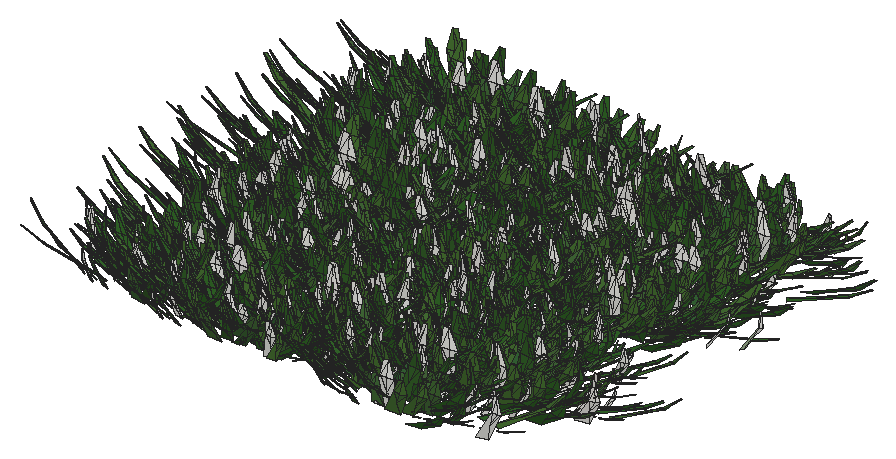
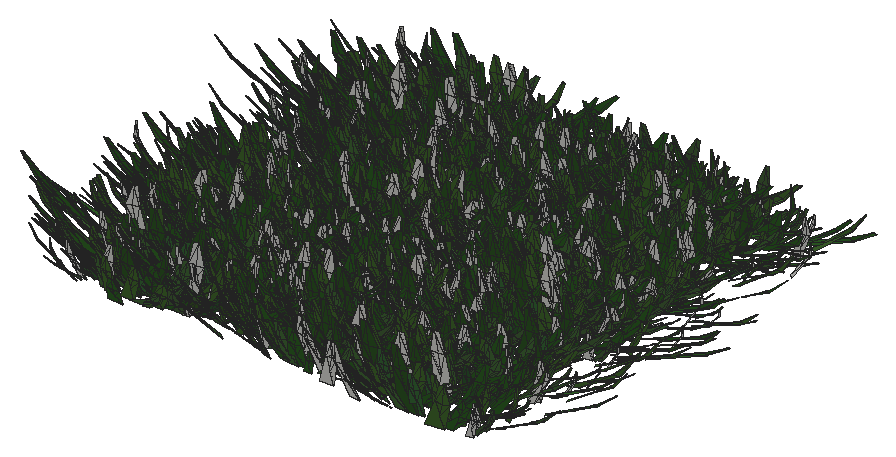
# SketchUp Ruby script. Lengths in inches.
U = 1.inch
M = Sketchup.active_model
def pt(a) = Geom::Point3d.new(a.map { |v| v * U })
def face(e, loops, mat)
  f = e.add_face(loops[0].map { |a| pt(a) })
  loops[1..].each { |l| e.add_face(l.map { |a| pt(a) }).erase! }
  f.material = f.back_material = mat if mat
  f
end
# faces: each face lists its corners as indices into pts; further lists are holes
def faces(e, pts, list, mat = nil) = list.each { |f| face(e, (f[0].is_a?(Array) ? f : [f]).map { |l| l.map { |i| pts[i] } }, mat) }
# xy, xz, yz: faces in a plane at the given z, y or x. An outline is a flat list of corners, or four numbers for a rectangle; further outlines are holes
def ring(l) = l.size == 4 ? [[l[0], l[1]], [l[2], l[1]], [l[2], l[3]], [l[0], l[3]]] : l.each_slice(2).to_a
def flat(e, list, mat, &to3) = list.each { |f| face(e, (f[0].is_a?(Array) ? f : [f]).map { |l| ring(l).map { |u, v| to3.(u, v) } }, mat) }
def xy(e, z, list, mat = nil) = flat(e, list, mat) { |x, y| [x, y, z] }
def xz(e, y, list, mat = nil) = flat(e, list, mat) { |x, z| [x, y, z] }
def yz(e, x, list, mat = nil) = flat(e, list, mat) { |y, z| [x, y, z] }
def lines(e, pts, list) = list.each { |a, b| e.add_line(pt(pts[a]), pt(pts[b])) }
# prism: a flat outline (further loops are holes) pulled along v
def prism(e, loops, v, mat = nil)
  f = face(e, loops, mat); d = Geom::Vector3d.new(v.map { |x| x * U })
  f.pushpull(f.normal.samedirection?(d) ? d.length : -d.length)
end
def box(e, o, s, mat = nil) = prism(e, [[o, [o[0] + s[0], o[1], o[2]], [o[0] + s[0], o[1] + s[1], o[2]], [o[0], o[1] + s[1], o[2]]]], [0, 0, s[2]], mat)
def at(x, y, z, deg = 0) = Geom::Transformation.translation(pt([x, y, z])) * Geom::Transformation.rotation(ORIGIN, Z_AXIS, deg.degrees)
def axes(o, x, y, z) = Geom::Transformation.new([*x, 0, *y, 0, *z, 0, *pt(o).to_a, 1])
def part(name) = M.definitions.add(name)
# library, detail: a bought-in or finely detailed component or shape, given as its bounding box
def library(name, o, s) = part(name).tap { |d| box(d.entities, o, s) }
def detail(e, o, s) = box(e.add_group.entities, o, s)
def put(e, d, t, mat = nil) = e.add_instance(d, t).tap { |i| i.material = mat if mat }
def group(e, t, mat = nil) = e.add_group.tap { |g| g.transformation = t; g.material = mat if mat }.entities
root = M.entities
M.materials.add("Material10").color = [48, 100, 38]
M.materials.add("Material3").color = [68, 110, 58]
M.materials.add("Material4").color = [48, 90, 38]
M.materials.add("Material5").color = [68, 110, 48]
M.materials.add("Material6").color = [48, 90, 48]
M.materials.add("Material7").color = [58, 110, 58]
M.materials.add("Material8").color = [58, 90, 38]
M.materials.add("Material9").color = [68, 100, 58]
c1 = part("grass00")
p = [[-0.6875,0.15,0],[-0.56,0.08,5.52],[-0.04,0.03,2.76],[0.48,-0.02,0],[0.35,-0.02,5.52],[-0.1,-0.14,5.52],
  [-0.12,0.65,8.37],[-0.42,0.65,8.37]]
faces(c1.entities,p,[[0,1,2,3],[3,2,4],[1,5,2],[5,4,2],[1,6,5],[4,5,6],[7,6,1]])
c2 = part("Group16\#1")
put(c2.entities,c1,axes([1.44,-0.61,-0.01],[0.05352,0.12609,0],[-0.10704,0.04543,0.07239],[0.06664,-0.02828,0.11628]),"Material6")
put(c2.entities,c1,axes([0.76,-0.15,-0.01],[0.04676,0.24062,0],[-0.23162,0.04501,0.06642],[0.0652,-0.01267,0.23595]),"Material3")
put(c2.entities,c1,axes([0.79,0.01,-0.01],[-0.00606,0.34651,0],[-0.34381,-0.00602,0.0432],[0.04319,0.00076,0.34386]))
put(c2.entities,c1,axes([1,0.23,-0.01],[-0.07192,0.31144,0],[-0.28722,-0.06632,0.1236],[0.12043,0.02781,0.29478]),"Material5")
put(c2.entities,c1,axes([1.66,0.77,-0.01],[-0.13828,0.29651,0],[-0.21551,-0.1005,0.22471],[0.20365,0.09498,0.23779]),"Material10")
put(c2.entities,c1,axes([0.6875,0.52,-0.01],[-0.18126,0.24051,0],[-0.22746,-0.17142,0.09788],[0.07817,0.05891,0.28481]),"Material5")
put(c2.entities,c1,axes([0.68,0.78,-0.01],[-0.215,0.18688,0],[-0.12385,-0.14248,0.21334],[0.13995,0.16101,0.18878]),"Material3")
put(c2.entities,c1,axes([0.56,1,-0.01],[-0.13756,0.07624,0],[-0.06159,-0.11112,0.0927],[0.04494,0.08108,0.12705]),"Material5")
put(c2.entities,c1,axes([0.2,0.64,-0.01],[-0.23729,0.07254,0],[-0.05711,-0.18681,0.153],[0.04473,0.14632,0.19535]),"Material10")
put(c2.entities,c1,axes([0.0625,0.72,-0.01],[-0.28874,0.02525,0],[-0.02179,-0.24916,0.14647],[0.01276,0.14591,0.25012]),"Material3")
put(c2.entities,c1,axes([-0.08,0.62,-0.01],[-0.34089,-0.04187,0],[0.03255,-0.26504,0.216],[-0.02633,0.21439,0.26703]),"Material10")
put(c2.entities,c1,axes([-0.34,0.98,-0.01],[-0.14314,-0.0493,0],[0.04397,-0.12769,0.06843],[-0.02228,0.0647,0.13505]),"Material10")
put(c2.entities,c1,axes([-0.87,1.45,-0.01],[-0.23488,-0.14114,0],[0.13761,-0.22901,0.06087],[-0.03135,0.05217,0.26717]))
put(c2.entities,c1,axes([-0.72,0.77,-0.01],[-0.14208,-0.13251,0],[0.07209,-0.0773,0.16301],[-0.11118,0.11922,0.1057]),"Material10")
put(c2.entities,c1,axes([-0.62,0.43,-0.01],[-0.14845,-0.21203,0],[0.18654,-0.13061,0.12304],[-0.10079,0.07057,0.22772]),"Material3")
put(c2.entities,c1,axes([-0.68,0.29,-0.01],[-0.13639,-0.32136,0],[0.31723,-0.13464,0.05579],[-0.05136,0.0218,0.34462]),"Material4")
put(c2.entities,c1,axes([-0.64,0.125,-0.01],[-0.0458,-0.23569,0],[0.22124,-0.043,0.08276],[-0.08124,0.01579,0.22538]),"Material7")
put(c2.entities,c1,axes([-1.6,-0.03,-0.01],[0.00576,-0.32897,0],[0.27526,0.00482,0.18018],[-0.18015,-0.00315,0.2753]),"Material5")
put(c2.entities,c1,axes([-1.36,-0.31,-0.01],[0.05718,-0.24765,0],[0.18172,0.04196,0.17267],[-0.16825,-0.03885,0.1865]),"Material10")
put(c2.entities,c1,axes([-1.54,-0.72,-0.01],[0.06537,-0.14017,0],[0.13555,0.06321,0.03939],[-0.0357,-0.01665,0.14956]))
put(c2.entities,c1,axes([-1.19,-0.9,-0.01],[0.09597,-0.12735,0],[0.11214,0.08451,0.07557],[-0.06035,-0.04548,0.14042]),"Material9")
put(c2.entities,c1,axes([-0.47,-0.54,-0.01],[0.11588,-0.10072,0],[0.0618,0.0711,0.12124],[-0.07953,-0.0915,0.0942]))
put(c2.entities,c1,axes([-0.47,-0.84,-0.01],[0.11927,-0.0661,0],[0.06603,0.11913,0.00646],[-0.00313,-0.00565,0.13621]),"Material5")
put(c2.entities,c1,axes([-0.38,-1.24,-0.01],[0.28037,-0.08571,0],[0.0618,0.20215,0.20315],[-0.05939,-0.19428,0.21139]),"Material9")
put(c2.entities,c1,axes([-0.06,-0.66,-0.01],[0.22719,-0.01987,0],[0.01247,0.14255,0.17758],[-0.01547,-0.17691,0.1431]),"Material8")
put(c2.entities,c1,axes([0.11,-0.89,-0.01],[0.14882,0.01828,0],[-0.01058,0.08611,0.12229],[0.01491,-0.12138,0.08676]),"Material6")
put(c2.entities,c1,axes([0.25,-0.72,-0.01],[0.20481,0.07053,0],[-0.06206,0.18022,0.10291],[0.03351,-0.0973,0.1906]),"Material6")
put(c2.entities,c1,axes([0.85,-1.42,-0.01],[0.16481,0.09904,0],[-0.09472,0.15762,0.05616],[0.02893,-0.04814,0.18389]),"Material5")
put(c2.entities,c1,axes([1.01,-1.09,-0.01],[0.21858,0.20385,0],[-0.17495,0.1876,0.15339],[0.10462,-0.11218,0.25652]),"Material10")
put(c2.entities,c1,axes([1.01,-0.71,-0.01],[0.08733,0.12473,0],[-0.06445,0.04512,0.13037],[0.1068,-0.07477,0.07867]),"Material6")
c3 = part("Group15\#1")
put(c3.entities,c2,at(0,0,0))
c4 = part("3darcstudiotree_grass00\#1")
put(c4.entities,c3,at(0,0,0))
put(root,c4,axes([60.36,24.12,7.6],[4.14217,-0.13896,0],[0.55231,1.029,-0.04419],[0.03401,0.06336,1.50171]))
put(root,c4,axes([61.51,38.26,7.6],[-3.78089,0.19176,0],[-0.79047,-0.97412,-0.01756],[-0.02482,-0.03059,1.76676]))
put(root,c4,axes([60.24,5.63,7.6],[3.46429,0.31864,0],[-1.65951,1.12765,-0.05896],[-0.1317,0.08949,1.94308]))
put(root,c4,axes([61.51,41.64,7.6],[0.85917,-1.09149,0],[4.23857,0.20853,-0.05061],[0.35882,0.01765,1.95081]))
put(root,c4,axes([62.11,26.89,7.6],[-4.66063,0.03187,0],[-0.11925,-1.09003,-0.04984],[-0.00747,-0.06831,1.49526]))
put(root,c4,axes([62.08,27.74,7.6],[0.72703,-1.03791,0],[5.00906,0.2193,-0.04237],[0.25355,0.0111,1.93074]))
put(root,c4,axes([61.48,22.57,7.6],[-2.37788,0.70827,0],[-3.16948,-0.66506,-0.02769],[-0.12287,-0.02578,1.49833]))
put(root,c4,axes([61.58,17.12,7.6],[-1.33257,1.11257,0],[-3.55566,-0.26617,-0.04102],[-0.28293,-0.02118,1.67021]))
put(root,c4,axes([62.17,16.2,7.6],[-3.55507,0.28812,0],[-1.24707,-0.96172,-0.02033],[-0.04772,-0.0368,1.92362]))
put(root,c4,axes([61.1875,35.42,7.6],[4.13598,0.19347,0],[-0.75584,1.00989,-0.00485],[-0.0061,0.00815,1.75633]))
put(root,c4,axes([61.05,9.8,7.6],[0.77095,1.02886,0],[-4.76297,0.22306,-0.00799],[-0.0391,0.00183,1.50733]))
put(root,c4,axes([61.85,19.33,7.6],[4.78466,-0.38044,0],[1.18012,0.92761,-0.00335],[0.00607,0.00477,1.45436]))
put(root,c4,axes([62.82,43.23,7.6],[1.77249,-0.83828,0],[4.36469,0.5768,-0.05061],[0.28357,0.03747,1.95538]))
put(root,c4,axes([63.67,6.61,7.6],[-4.81545,-0.2901,0],[1.06341,-1.10323,-0.03666],[0.0394,-0.04088,1.30149]))
put(root,c4,axes([64,11.27,7.6],[-3.36311,-0.90745,0],[3.5657,-0.82593,-0.02123],[0.07378,-0.01709,1.43939]))
put(root,c4,axes([62.4,29.69,7.6],[4.34926,-0.09263,0],[0.33262,0.97608,-0.01096],[0.00735,0.02158,1.93666]))
put(root,c4,axes([63.82,34.02,7.6],[1.03751,-0.98763,0],[4.08479,0.26819,-0.03356],[0.19811,0.01301,1.61101]))
put(root,c4,axes([62.71,12.97,7.6],[4.36652,-0.10456,0],[0.38952,1.01663,-0.02913],[0.02165,0.05651,1.9903]))
put(root,c4,axes([64.2,25.04,7.6],[0.12365,-1.27532,0],[4.95988,0.03006,-0.04883],[0.25094,0.00152,1.59403]))
put(root,c4,axes([62.38,20.43,7.6],[1.52464,0.86954,0],[-4.15594,0.45544,-0.01361],[-0.07039,0.00771,1.60179]))
put(root,c4,axes([63.23,32.51,7.6],[4.76541,-0.43818,0],[1.55968,1.06014,-0.01984],[0.0463,0.03147,1.90869]))
put(root,c4,axes([63.68,36.97,7.6],[3.07982,0.93534,0],[-3.08003,0.63386,-0.01155],[-0.0607,0.01249,1.69697]))
put(root,c4,axes([66.08,18.09,7.6],[-3.49123,-0.27922,0],[1.51464,-1.18364,-0.00535],[0.00882,-0.00689,1.67969]))
put(root,c4,axes([66.24,24,7.6],[0.13314,-1.12565,0],[4.81374,0.03558,-0.0158],[0.0905,0.00067,1.72451]))
put(root,c4,axes([66.53,10.14,7.6],[0.0625,-0.92457,0],[5.11457,0.02161,-0.02351],[0.11863,0.0005,1.61343]))
put(root,c4,axes([65.87,15.59,7.6],[2.8016,-0.76743,0],[3.52577,0.80446,-0.03913],[0.15024,0.03428,1.55084]))
put(root,c4,axes([66.61,27.98,7.6],[-5.10128,0.24176,0],[-0.82054,-1.08211,-0.04366],[-0.05047,-0.06656,1.70895]))
put(root,c4,axes([66.96,22.38,7.6],[-4.96044,-0.06591,0],[0.25075,-1.17948,-0.02618],[0.00816,-0.03838,1.73378]))
put(root,c4,axes([67.33,35.67,7.6],[-3.94461,-0.5014,0],[1.7984,-0.88427,-0.05096],[0.14967,-0.07359,1.60728]))
put(root,c4,axes([65.98,34.6,7.6],[3.7762,-0.18672,0],[0.72842,0.92072,-0.00259],[0.00364,0.0046,1.70099]))
put(root,c4,axes([66.33,31.47,7.6],[3.67314,-0.43874,0],[1.76522,0.92366,-0.01719],[0.04935,0.02582,1.70421]))
put(root,c4,axes([67.75,39.09,7.6],[-3.93857,-0.30978,0],[1.37085,-1.08932,-0.00258],[0.00367,-0.00291,1.35273]))
put(root,c4,axes([68.09,11.4375,7.6],[-3.44755,-0.92992,0],[3.38069,-0.78334,-0.01903],[0.09302,-0.02155,1.91973]))
put(root,c4,axes([66.99,18.61,7.6],[-2.366,0.989,0],[-3.30831,-0.49466,-0.01081],[-0.05313,-0.00794,1.38013]))
put(root,c4,axes([67.5,41.79,7.6],[2.17212,-0.7546,0],[4.09706,0.73708,-0.05142],[0.26111,0.04697,1.97373]))
put(root,c4,axes([66.51,20.67,7.6],[2.16605,0.76484,0],[-3.80323,0.67318,-0.06047],[-0.22732,0.04024,1.34144]))
put(root,c4,axes([68.42,37.48,7.6],[-1.30769,-0.93335,0],[3.48924,-0.30554,-0.02961],[0.16247,-0.01423,1.34337]))
put(root,c4,axes([67.46,14.66,7.6],[-1.89044,1.0999,0],[-3.63234,-0.39019,-0.02574],[-0.12693,-0.01363,1.32606]))
put(root,c4,axes([67.45,26.95,7.6],[3.25343,-0.44268,0],[1.93711,0.88978,-0.04084],[0.14968,0.06875,1.94165]))
put(root,c4,axes([69.23,29.77,7.6],[-2.99003,-0.56506,0],[2.79267,-0.92359,-0.03674],[0.12403,-0.04102,1.62045]))
put(root,c4,axes([69.23,8.03,7.6],[-4.96013,0.01619,0],[-0.06304,-1.20724,-0.02897],[-0.0018,-0.03442,1.4344]))
put(root,c4,axes([67.97,39.8,7.6],[3.80777,-0.2002,0],[0.96857,1.15138,-0.04208],[0.03932,0.04675,1.3356]))
put(root,c4,axes([67.88,5.97,7.6],[3.481,0.74238,0],[-3.25262,0.95321,-0.05603],[-0.20851,0.06111,1.79617]))
put(root,c4,axes([69.37,13.11,7.6],[-3.23012,0.53983,0],[-2.03325,-0.76039,-0.00767],[-0.03049,-0.0114,1.63569]))
put(root,c4,axes([69.7,33.16,7.6],[1.70325,-1.05974,0],[4.66988,0.4691,-0.03894],[0.22464,0.02257,1.95573]))
put(root,c4,axes([69.53,25.52,7.6],[2.4144,-1.08588,0],[3.3917,0.47133,-0.02727],[0.14209,0.01975,1.44583]))
put(root,c4,axes([68.93,6.75,7.6],[4.57432,-0.02417,0],[0.10814,1.27933,-0.00824],[0.00087,0.0103,1.59977]))
put(root,c4,axes([69.38,4.33,7.6],[4.10387,0.33855,0],[-1.15114,0.87212,-0.0401],[-0.09251,0.07009,1.69032]))
put(root,c4,axes([71.99,29.92,7.6],[-4.98676,0.19311,0],[-0.7421,-1.19771,-0.03016],[-0.02479,-0.04002,1.62739]))
put(root,c4,axes([73.03,20.97,7.6],[-1.79404,-0.94481,0],[3.82512,-0.45395,-0.00409],[0.0193,-0.00229,1.3842]))
put(root,c4,axes([72.42,5.19,7.6],[-3.73442,0.23061,0],[-0.95038,-0.96187,-0.03348],[-0.04929,-0.04988,1.52035]))
put(root,c4,axes([72.89,21.68,7.6],[2.59296,-0.87117,0],[4.05566,0.75445,-0.00846],[0.02997,0.00558,1.39582]))
put(root,c4,axes([73.77,38.4,7.6],[-4.85,-0.22958,0],[0.83383,-1.10092,-0.02653],[0.02986,-0.03943,1.69452]))
put(root,c4,axes([73.76,16.42,7.6],[-3.94716,-0.15767,0],[0.6625,-1.03659,-0.01241],[0.00983,-0.01538,1.31731]))
put(root,c4,axes([72.55,24.99,7.6],[4.34642,-0.40872,0],[1.45862,0.96946,-0.01237],[0.03108,0.02066,1.84855]))
put(root,c4,axes([74.2,7.96,7.6],[-4.3345,-0.18054,0],[0.62418,-0.93658,-0.01531],[0.0191,-0.02866,1.80136]))
put(root,c4,axes([74.04,10.92,7.6],[1.02924,-1.1219,0],[3.76479,0.21587,-0.013],[0.10318,0.00592,1.96601]))
put(root,c4,axes([74.49,13.13,7.6],[-1.06084,-1.17828,0],[4.37174,-0.246,-0.03143],[0.16722,-0.00941,1.52743]))
put(root,c4,axes([74.82,28.58,7.6],[-1.72294,-1.06651,0],[4.16754,-0.42079,-0.01424],[0.06745,-0.00681,1.43479]))
put(root,c4,axes([74.66,39.85,7.6],[-3.78747,-0.21466,0],[0.95822,-1.0567,-0.03754],[0.05955,-0.06567,1.94323]))
put(root,c4,axes([74.34,14.06,7.6],[-0.48134,-1.10906,0],[3.87122,-0.10501,-0.05057],[0.36681,-0.00995,1.77563]))
put(root,c4,axes([73.23,23.59,7.6],[3.37993,0.45978,0],[-1.93327,0.88823,-0.04213],[-0.10808,0.04966,1.35679]))
put(root,c4,axes([74.55,10.36,7.6],[3.21509,-0.82009,0],[3.01925,0.73979,-0.0131],[0.0637,0.01561,1.79861]))
put(root,c4,axes([75.48,30.62,7.6],[-3.80165,-0.22525,0],[1.19413,-1.25962,-0.00987],[0.01044,-0.01102,1.48448]))
put(root,c4,axes([73.49,19.04,7.6],[3.93668,0.7746,0],[-2.90323,0.92217,-0.01986],[-0.08093,0.02571,1.93312]))
put(root,c4,axes([74.39,7.09,7.6],[-0.79276,1.18933,0],[-3.59183,-0.14964,-0.00349],[-0.02047,-0.00085,1.35435]))
put(root,c4,axes([74.4,43.01,7.6],[4.30418,0.00494,0],[-0.017,0.92497,-0.03904],[-0.00144,0.07818,1.85207]))
put(root,c4,axes([75.5,17,7.6],[2.16099,-1.18023,0],[3.73882,0.42786,-0.04178],[0.24002,0.02747,1.62381]))
put(root,c4,axes([74.5625,26.15,7.6],[3.61999,0.64217,0],[-2.78348,0.98067,-0.05586],[-0.16431,0.05789,1.52805]))
put(root,c4,axes([75.58,37.33,7.6],[3.39209,-0.30668,0],[1.53109,1.05845,-0.04794],[0.07887,0.05453,1.36124]))
put(root,c4,axes([76.4,36.27,7.6],[3.28078,-0.54762,0],[2.6685,0.99917,-0.03164],[0.11118,0.04163,1.90074]))
put(root,c4,axes([76,41.43,7.6],[4.6588,-0.38386,0],[1.34446,1.01982,-0.0158],[0.03633,0.02756,1.97161]))
put(root,c4,axes([75.625,34.56,7.6],[1.88884,1.20061,0],[-4.32214,0.42498,-0.01805],[-0.11016,0.01083,1.90362]))
put(root,c4,axes([76.23,32.34,7.6],[4.87019,-0.36873,0],[1.38522,1.1435,-0.03542],[0.04951,0.04087,1.44036]))
put(root,c4,axes([78.15,20.7,7.6],[-3.20652,-0.59771,0],[2.76266,-0.9263,-0.01853],[0.05834,-0.01956,1.52144]))
put(root,c4,axes([78.47,28.7,7.6],[-4.04993,-0.77594,0],[2.93522,-0.9575,-0.01589],[0.04448,-0.01451,1.38765]))
put(root,c4,axes([78.11,32.58,7.6],[-4.54229,0.0918,0],[-0.30554,-0.94485,-0.02584],[-0.01532,-0.04736,1.74304]))
put(root,c4,axes([77.99,37.32,7.6],[2.61594,-0.62324,0],[2.61447,0.68586,-0.03437],[0.16704,0.04382,1.66865]))
put(root,c4,axes([78.76,40.17,7.6],[0.42125,-1.19943,0],[4.10961,0.09021,-0.02351],[0.14993,0.00329,1.65028]))
put(root,c4,axes([78.09,17.46,7.6],[3.29935,0.67285,0],[-2.48006,0.76006,-0.0073],[-0.03648,0.01118,1.93831]))
put(root,c4,axes([80.25,41.24,7.6],[-4.60962,0.0959,0],[-0.32649,-0.98088,-0.01346],[-0.00781,-0.02346,1.72106]))
put(root,c4,axes([80.52,8.36,7.6],[-3.45897,-0.26737,0],[1.38281,-1.1181,-0.02785],[0.05102,-0.04126,1.81462]))
put(root,c4,axes([79.79,11.58,7.6],[-1.6569,0.8411,0],[-3.67968,-0.45304,-0.03193],[-0.19007,-0.0234,1.70102]))
put(root,c4,axes([81.03,16.01,7.6],[-4.11024,0.08918,0],[-0.31404,-0.9046,-0.03872],[-0.02635,-0.07591,1.78675]))
put(root,c4,axes([79.99,12.98,7.6],[3.52313,0.28357,0],[-1.27249,0.9881,-0.048],[-0.10422,0.08093,1.83855]))
put(root,c4,axes([81.52,38.68,7.6],[1.09083,-0.85917,0],[4.87884,0.38714,-0.04397],[0.18771,0.0149,1.43296]))
put(root,c4,axes([82.36,23.92,7.6],[-1.14436,-0.88187,0],[4.48808,-0.364,-0.01227],[0.07282,-0.00591,1.83962]))
put(root,c4,axes([81.875,35.79,7.6],[1.53749,-0.92212,0],[4.0104,0.41792,-0.02113],[0.10884,0.01134,1.51549]))
put(root,c4,axes([80.29,29.62,7.6],[1.39417,1.1395,0],[-4.86141,0.37174,-0.03143],[-0.13527,0.01034,1.42994]))
put(root,c4,axes([81.08,24.6,7.6],[4.06384,-0.63322,0],[2.31994,0.93055,-0.04378],[0.15154,0.06078,1.79394]))
put(root,c4,axes([80.75,26.25,7.6],[3.66016,0.09208,0],[-0.4718,1.17207,-0.00091],[-0.00045,0.00113,1.45853]))
put(root,c4,axes([80.64,19.17,7.6],[0.81023,1.10626,0],[-4.8699,0.22292,-0.04305],[-0.25037,0.01146,1.82947]))
put(root,c4,axes([80.8,7.45,7.6],[3.47121,0.32425,0],[-1.57021,1.05061,-0.02415],[-0.05805,0.03884,1.92547]))
put(root,c4,axes([81.125,21.85,7.6],[0.63588,1.22934,0],[-4.27821,0.13831,-0.04685],[-0.28868,0.00933,1.67517]))
put(root,c4,axes([82.43,30.94,7.6],[1.12622,-0.91153,0],[3.70574,0.28616,-0.03395],[0.20191,0.01559,1.50895]))
put(root,c4,axes([81.36,5.8,7.6],[3.08399,0.48066,0],[-1.99021,0.79809,-0.0044],[-0.01295,0.00519,1.30779]))
put(root,c4,axes([81.37,34.0625,7.6],[3.86594,0.83132,0],[-2.86233,0.83193,-0.04839],[-0.1699,0.04938,1.47711]))
put(root,c4,axes([81.49,9.61,7.6],[3.60165,0.48715,0],[-2.30784,1.06642,-0.00222],[-0.0056,0.00259,1.6055]))
put(root,c4,axes([82.03,14.61,7.6],[3.64912,0.26405,0],[-1.21989,1.05365,-0.02015],[-0.03346,0.0289,1.63787]))
put(root,c4,axes([84.74,17.69,7.6],[-2.66703,-0.80905,0],[2.89138,-0.59571,-0.03867],[0.19078,-0.03931,1.49724]))
put(root,c4,axes([85.18,38.33,7.6],[-2.83131,-0.59353,0],[3.0716,-0.91578,-0.0116],[0.03498,-0.01043,1.40225]))
put(root,c4,axes([85.31,20.35,7.6],[-3.90478,-0.61757,0],[2.54983,-1.00763,-0.01513],[0.04881,-0.01929,1.79885]))
put(root,c4,axes([85.17,7.43,7.6],[-3.22402,-0.42801,0],[2.1572,-1.01557,-0.05452],[0.12489,-0.05879,1.404]))
put(root,c4,axes([84.07,32.28,7.6],[3.49835,-0.41383,0],[1.60405,0.84749,-0.01286],[0.03427,0.0181,1.45976]))
put(root,c4,axes([84.57,11.32,7.6],[-4.05846,0.5498,0],[-2.41739,-1.11529,-0.0133],[-0.0389,-0.01795,1.94738]))
put(root,c4,axes([85.26,4.1,7.6],[0.61281,-1.25792,0],[4.16429,0.12679,-0.0324],[0.1815,0.00553,1.47946]))
put(root,c4,axes([84.47,29.78,7.6],[-0.28726,1.27917,0],[-3.62125,-0.05083,-0.00552],[-0.03584,-0.0005,1.47331]))
put(root,c4,axes([86.28,9.63,7.6],[1.5261,-1.19927,0],[4.79938,0.38171,-0.00448],[0.02429,0.00193,1.79011]))
put(root,c4,axes([86.04,12.45,7.6],[-0.47435,-1.1855,0],[4.17095,-0.10431,-0.05423],[0.34983,-0.00875,1.69842]))
put(root,c4,axes([86.37,28.47,7.6],[-3.66287,-0.10914,0],[0.53272,-1.11739,-0.01308],[0.00905,-0.01898,1.64432]))
put(root,c4,axes([86.48,37.0625,7.6],[-4.43451,0.03772,0],[-0.16554,-1.21627,-0.01213],[-0.00253,-0.01859,1.86653]))
put(root,c4,axes([86.33,21.57,7.6],[-3.65887,0.1299,0],[-0.61787,-1.08767,-0.00819],[-0.00564,-0.00993,1.3463]))
put(root,c4,axes([86.13,14.97,7.6],[-3.669,0.60681,0],[-2.27303,-0.85898,-0.03289],[-0.10969,-0.04145,1.55622]))
put(root,c4,axes([87.03,41.32,7.6],[-4.28497,-0.45872,0],[1.95501,-1.14138,-0.00601],[0.01191,-0.00695,1.5624]))
put(root,c4,axes([86.93,18.63,7.6],[-3.05739,-0.71664,0],[2.47729,-0.66055,-0.04465],[0.23187,-0.06183,1.71883]))
put(root,c4,axes([87.41,5.02,7.6],[-4.36075,-0.60413,0],[2.40015,-1.0828,-0.02403],[0.07228,-0.03261,1.92026]))
put(root,c4,axes([85.12,25.5,7.6],[3.04221,0.50388,0],[-2.77722,1.04797,-0.00365],[-0.00864,0.00326,1.34685]))
put(root,c4,axes([86.02,35.4,7.6],[4.61314,0.2073,0],[-0.8279,1.1515,-0.00017],[-0.00019,0.00026,1.78268]))
put(root,c4,axes([87.78,8.41,7.6],[-2.44705,-0.6793,0],[3.03744,-0.68387,-0.04825],[0.26014,-0.05857,1.85346]))
put(root,c4,axes([87,33.87,7.6],[-2.92283,0.91805,0],[-3.29129,-0.65491,-0.02078],[-0.1142,-0.02272,1.84714]))
put(root,c4,axes([86.16,15.95,7.6],[4.43029,0.19931,0],[-0.91399,1.26978,-0.01866],[-0.01759,0.02444,1.717]))
put(root,c4,axes([86.51,31.05,7.6],[3.52512,0.8325,0],[-3.53899,0.93659,-0.01632],[-0.05093,0.01348,1.46423]))
put(root,c4,axes([87,26.1,7.6],[3.74573,0.67429,0],[-2.32637,0.8077,-0.02682],[-0.11092,0.03851,1.76121]))
put(root,c4,axes([88.37,40.32,7.6],[-1.7815,0.94038,0],[-4.05374,-0.47998,-0.05633],[-0.34181,-0.04047,1.88219]))
put(root,c4,axes([88,23.91,7.6],[2.43331,0.85712,0],[-3.60269,0.63924,-0.0048],[-0.0225,0.00399,1.58899]))
put(root,c4,axes([90.17,14.52,7.6],[-3.5004,-0.31733,0],[1.33107,-0.91766,-0.00444],[0.00863,-0.00595,1.39182]))
put(root,c4,axes([90.97,32.33,7.6],[0.98634,-0.98273,0],[4.96113,0.31121,-0.03647],[0.15012,0.00942,1.35653]))
put(root,c4,axes([90.85,41.73,7.6],[1.5516,-0.99587,0],[4.11909,0.4011,-0.0174],[0.07644,0.00744,1.30214]))
put(root,c4,axes([90.77,23.83,7.6],[1.28741,-1.026,0],[3.77436,0.296,-0.02865],[0.19326,0.01516,1.74795]))
put(root,c4,axes([90.38,13.43,7.6],[2.57556,-0.96136,0],[3.42516,0.57352,-0.05113],[0.25858,0.0433,1.56833]))
put(root,c4,axes([91.4,10.13,7.6],[0.62856,-1.17531,0],[4.83812,0.16171,-0.0102],[0.05862,0.00196,1.76846]))
put(root,c4,axes([91.72,17.85,7.6],[-3.61051,-0.41144,0],[1.52061,-0.83398,-0.0331],[0.09259,-0.05078,1.54531]))
put(root,c4,axes([90.46,15.61,7.6],[2.93142,0.86988,0],[-2.89804,0.61038,-0.04423],[-0.19713,0.04152,1.38013]))
put(root,c4,axes([91.71,31.51,7.6],[2.02846,-0.79273,0],[3.7574,0.60091,-0.02581],[0.12575,0.02011,1.61243]))
put(root,c4,axes([92.26,25.14,7.6],[-0.79202,-1.12645,0],[4.16541,-0.18305,-0.04893],[0.31505,-0.01384,1.72817]))
put(root,c4,axes([91.97,40.23,7.6],[-4.0818,0.563,0],[-2.02545,-0.91779,-0.01481],[-0.0392,-0.01776,1.43556]))
put(root,c4,axes([91.26,34.4375,7.6],[4.56829,-0.12289,0],[0.55043,1.27888,-0.03237],[0.01647,0.03827,1.52951]))
put(root,c4,axes([92.94,11.61,7.6],[-4.66423,-0.46806,0],[1.3813,-0.8603,-0.04034],[0.1029,-0.06409,1.58691]))
put(root,c4,axes([92.875,29.52,7.6],[-0.8253,-1.0659,0],[3.55539,-0.17205,-0.00678],[0.0454,-0.0022,1.54322]))
put(root,c4,axes([93.38,26.97,7.6],[-2.41791,-1.09567,0],[4.13972,-0.57097,-0.0117],[0.05943,-0.0082,1.7149]))
put(root,c4,axes([91.62,42.81,7.6],[1.31705,0.88702,0],[-3.52607,0.32722,-0.04291],[-0.24696,0.02292,1.44315]))
put(root,c4,axes([92.47,37.81,7.6],[2.84794,-0.83805,0],[3.51838,0.74728,-0.02612],[0.12969,0.02754,1.8801]))
